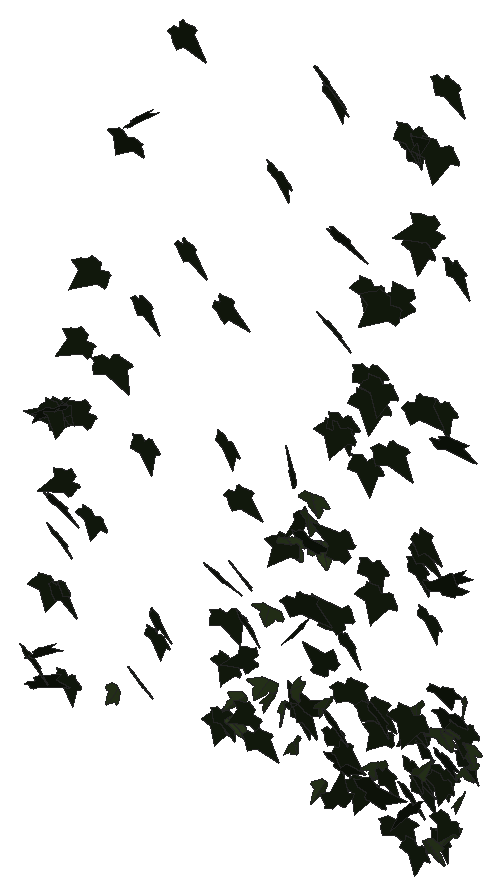
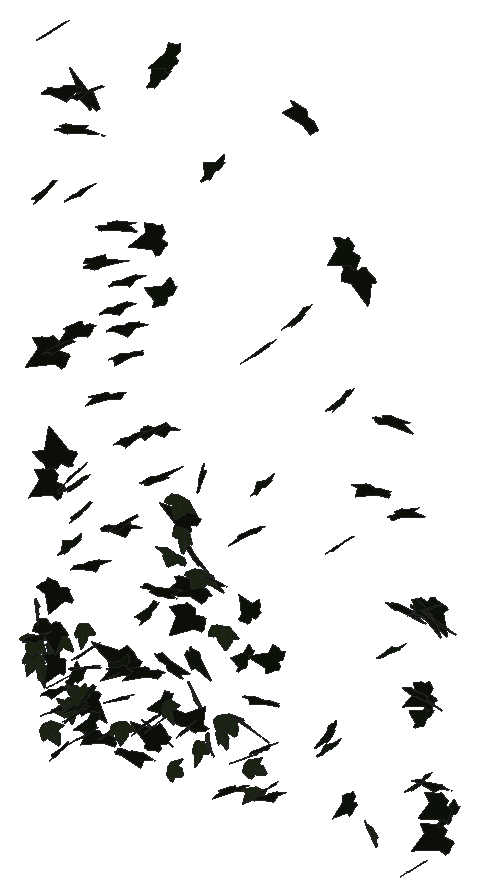
# SketchUp Ruby script. Lengths in inches.
U = 1.inch
M = Sketchup.active_model
def pt(a) = Geom::Point3d.new(a.map { |v| v * U })
def face(e, loops, mat)
  f = e.add_face(loops[0].map { |a| pt(a) })
  loops[1..].each { |l| e.add_face(l.map { |a| pt(a) }).erase! }
  f.material = f.back_material = mat if mat
  f
end
# faces: each face lists its corners as indices into pts; further lists are holes
def faces(e, pts, list, mat = nil) = list.each { |f| face(e, (f[0].is_a?(Array) ? f : [f]).map { |l| l.map { |i| pts[i] } }, mat) }
# xy, xz, yz: faces in a plane at the given z, y or x. An outline is a flat list of corners, or four numbers for a rectangle; further outlines are holes
def ring(l) = l.size == 4 ? [[l[0], l[1]], [l[2], l[1]], [l[2], l[3]], [l[0], l[3]]] : l.each_slice(2).to_a
def flat(e, list, mat, &to3) = list.each { |f| face(e, (f[0].is_a?(Array) ? f : [f]).map { |l| ring(l).map { |u, v| to3.(u, v) } }, mat) }
def xy(e, z, list, mat = nil) = flat(e, list, mat) { |x, y| [x, y, z] }
def xz(e, y, list, mat = nil) = flat(e, list, mat) { |x, z| [x, y, z] }
def yz(e, x, list, mat = nil) = flat(e, list, mat) { |y, z| [x, y, z] }
def lines(e, pts, list) = list.each { |a, b| e.add_line(pt(pts[a]), pt(pts[b])) }
# prism: a flat outline (further loops are holes) pulled along v
def prism(e, loops, v, mat = nil)
  f = face(e, loops, mat); d = Geom::Vector3d.new(v.map { |x| x * U })
  f.pushpull(f.normal.samedirection?(d) ? d.length : -d.length)
end
def box(e, o, s, mat = nil) = prism(e, [[o, [o[0] + s[0], o[1], o[2]], [o[0] + s[0], o[1] + s[1], o[2]], [o[0], o[1] + s[1], o[2]]]], [0, 0, s[2]], mat)
def at(x, y, z, deg = 0) = Geom::Transformation.translation(pt([x, y, z])) * Geom::Transformation.rotation(ORIGIN, Z_AXIS, deg.degrees)
def axes(o, x, y, z) = Geom::Transformation.new([*x, 0, *y, 0, *z, 0, *pt(o).to_a, 1])
def part(name) = M.definitions.add(name)
# library, detail: a bought-in or finely detailed component or shape, given as its bounding box
def library(name, o, s) = part(name).tap { |d| box(d.entities, o, s) }
def detail(e, o, s) = box(e.add_group.entities, o, s)
def put(e, d, t, mat = nil) = e.add_instance(d, t).tap { |i| i.material = mat if mat }
def group(e, t, mat = nil) = e.add_group.tap { |g| g.transformation = t; g.material = mat if mat }.entities
root = M.entities
M.materials.add("1026 AP 7946 SUNNY SIDE UP").color = [254, 231, 186]
M.materials.add("efeu1").color = [18, 25, 13]
M.materials.add("efeu2").color = [43, 57, 29]
c1 = part("ivyleaf_9")
p = [[1.54,2.16,1.25],[1.36,2.04,1.19],[-0.21,0.99,0.68],[-0.71,1.11,0.82],[-0.85,0.86,0.67],[-0.8,0.17,0.21],
  [-0.9,-0.01,0.1],[-0.67,-0.16,-0.02],[-0.08,-0.08,-0.05],[-0.03,-0.6,-0.4],[0.65,-0.88,-0.66],[0.83,-0.6,-0.49],
  [1.29,-0.42,-0.43],[1.8125,-0.07,-0.26],[1.21,0.44,0.15]]
faces(c1.entities,p,[[0,1,2,3,4,5,6,7,8,9,10,11,12,13,14]],"efeu1")
c2 = part("ivyleaf_10")
p = [[0,0.5,-0.03],[-0.0625,2.02,-0.43],[-0.19,2.01,-0.46],[-0.54,1.05,-0.29],[-0.52,0.625,-0.18],[-0.83,0.76,-0.28],
  [-1.16,0.64,-0.33],[-1.15,0.33,-0.24],[-0.77,-0.39,0.02],[-0.3,-0.51,0.16],[0.04,-0.48,0.23],[-0.02,2.01,-0.4375],
  [-0.06,2.01,-0.43],[0.04,-0.49,0.23],[0.67,-0.49,0.14],[1.38,0.36,-0.2],[1.375,0.51,-0.24],[0.81,0.65,-0.19],
  [0.62,0.59,-0.15],[0.6,1.09,-0.28],[0.5,1.23,-0.31]]
faces(c2.entities,p,[[0,1,2,3,4,5,6,7,8,9,10],[11,12,0,13,14,15,16,17,18,19,20]],"efeu2")
put(root,c1,axes([99.83,212.1875,300.87],[-0.58359,0.05469,0.08508],[-0.13611,-0.0259,-0.38471],[-0.07485,-0.37927,0.03627]),"1026 AP 7946 SUNNY SIDE UP")
put(root,c1,axes([99.74,211.14,304.6],[-0.03122,0.37574,-0.19386],[-0.0981,-0.18665,-0.4002],[-0.7049,0.00934,0.06428]),"1026 AP 7946 SUNNY SIDE UP")
put(root,c1,axes([99.41,211.6,296.37],[-0.47274,-0.25055,-0.10343],[0.23864,-0.02256,-0.38449],[0.38608,-0.29284,0.11101]),"1026 AP 7946 SUNNY SIDE UP")
put(root,c1,axes([100.02,211.4,304.22],[-0.5025,0.19094,0.23112],[-0.35056,0.07026,-0.37301],[-0.33673,-0.35808,0.04344]),"1026 AP 7946 SUNNY SIDE UP")
put(root,c1,axes([99.85,211.42,304.61],[-0.25238,0.37371,-0.02021],[-0.03373,-0.03339,-0.42979],[-0.63478,-0.14681,0.03087]),"1026 AP 7946 SUNNY SIDE UP")
put(root,c1,axes([99.59,211.3125,300.41],[0.62802,-0.14559,0.00543],[-0.01208,-0.03703,-0.4243],[0.24713,0.36817,-0.03454]),"1026 AP 7946 SUNNY SIDE UP")
put(root,c1,axes([99.82,211.47,304.43],[-0.215,-0.37216,0.08626],[0.03995,-0.09744,-0.41847],[0.64696,-0.11766,0.0545]),"1026 AP 7946 SUNNY SIDE UP")
put(root,c1,axes([99.62,209.84,293.97],[0.27049,-0.33274,0.17999],[0.10805,-0.16065,-0.39704],[0.62696,0.17124,-0.00923]),"1026 AP 7946 SUNNY SIDE UP")
put(root,c1,axes([99.73,211.52,296.33],[0.28251,-0.33441,-0.08104],[-0.03589,0.06913,-0.39873],[0.57933,0.16736,0.01482]),"1026 AP 7946 SUNNY SIDE UP")
put(root,c1,axes([99.99,211.83,292.19],[-0.00976,-0.3614,0.06],[0.00416,-0.0608,-0.38778],[0.62208,-0.00526,0.00354]),"1026 AP 7946 SUNNY SIDE UP")
put(root,c1,axes([100.01,209.74,294.23],[0.3581,0.22641,0.29105],[0.26971,0.21835,-0.3272],[-0.53232,0.26294,0.03001]),"1026 AP 7946 SUNNY SIDE UP")
put(root,c1,axes([99.94,209.9375,292.86],[0.47353,0.22274,0.23306],[0.29589,0.12583,-0.38028],[-0.434,0.32881,-0.00498]),"1026 AP 7946 SUNNY SIDE UP")
put(root,c1,axes([99.97,211.08,299.05],[0.21611,-0.29973,0.20391],[0.14768,-0.17645,-0.34057],[0.54667,0.16616,0.0114]),"1026 AP 7946 SUNNY SIDE UP")
put(root,c1,axes([100.86,211.91,304.47],[-0.6169,-0.0056,0.05529],[-0.08298,-0.04357,-0.4021],[0.01796,-0.39358,0.0414]),"1026 AP 7946 SUNNY SIDE UP")
put(root,c1,axes([101.42,211.07,308.3],[-0.41103,-0.22863,0.2234],[-0.23064,-0.16298,-0.35799],[0.44012,-0.29893,0.02103]),"1026 AP 7946 SUNNY SIDE UP")
put(root,c1,axes([102.57,210.5,312.17],[-0.60558,-0.15883,0.07956],[-0.0951,-0.05776,-0.42841],[0.26158,-0.38871,0.02845]),"1026 AP 7946 SUNNY SIDE UP")
put(root,c1,axes([102.45,210.375,300.97],[-0.15504,-0.33744,0.18943],[0.06958,-0.20044,-0.352],[0.60168,-0.06377,0.08952]),"1026 AP 7946 SUNNY SIDE UP")
put(root,c2,axes([102.84,211.22,292.86],[0.40782,-0.25476,-0.08],[-0.09027,0.05029,-0.37421],[0.40826,0.26561,-0.00283]),"1026 AP 7946 SUNNY SIDE UP")
put(root,c1,axes([103.41,210.25,308.45],[-0.15653,-0.3069,-0.27978],[0.34611,0.19373,-0.30951],[0.54139,-0.21258,0.11698]),"1026 AP 7946 SUNNY SIDE UP")
put(root,c1,axes([104,210.53,318.68],[0.39544,0.08936,-0.3623],[-0.50401,-0.14716,-0.27512],[-0.26908,0.40698,-0.01712]),"1026 AP 7946 SUNNY SIDE UP")
put(root,c1,axes([103.65,211.38,293.86],[0.49089,-0.18472,-0.10069],[-0.13516,0.04458,-0.3734],[0.29869,0.32376,-0.00349]),"1026 AP 7946 SUNNY SIDE UP")
put(root,c1,axes([104.34,210.55,319.54],[0.29308,0.24023,0.3354],[0.23971,0.28873,-0.309],[-0.58745,0.23767,0.04124]),"1026 AP 7946 SUNNY SIDE UP")
put(root,c1,axes([104.73,211.33,296.88],[0.401,-0.25528,-0.1437],[-0.16759,0.08854,-0.37102],[0.42445,0.27614,-0.01073]),"1026 AP 7946 SUNNY SIDE UP")
put(root,c1,axes([104.86,211.41,295.99],[-0.00841,-0.34617,0.16765],[0.05573,-0.16446,-0.35587],[0.6002,0.01042,0.03539]),"1026 AP 7946 SUNNY SIDE UP")
put(root,c1,axes([105.06,210.39,305.26],[0.02898,-0.41221,0.02212],[-0.00057,-0.02385,-0.42522],[0.64924,0.01838,-0.00136]),"1026 AP 7946 SUNNY SIDE UP")
put(root,c1,axes([105.22,209.9,311.93],[0.32539,-0.37606,-0.06268],[-0.0472,0.05049,-0.4419],[0.59662,0.20909,-0.00078]),"1026 AP 7946 SUNNY SIDE UP")
put(root,c1,axes([107.09,210.11,324.84],[-0.019,-0.13716,-0.46068],[0.71861,0.08836,-0.04019],[0.151,-0.43773,0.13332]),"1026 AP 7946 SUNNY SIDE UP")
put(root,c1,axes([107.4,209.93,315.23],[0.38057,-0.35202,-0.12857],[-0.08086,0.11349,-0.4389],[0.58063,0.24653,0.02315]),"1026 AP 7946 SUNNY SIDE UP")
put(root,c1,axes([107.25,211.89,299.55],[0.40144,-0.22967,0.20304],[0.25758,-0.11396,-0.35375],[0.40173,0.30258,0.02393]),"1026 AP 7946 SUNNY SIDE UP")
put(root,c1,axes([107.78,211.875,292.96],[-0.25651,-0.32362,0.03608],[-0.00352,-0.04011,-0.37322],[0.51213,-0.16237,0.0155]),"1026 AP 7946 SUNNY SIDE UP")
put(root,c1,axes([107.78,212.31,295.38],[-0.20276,-0.32363,0.12616],[-0.02449,-0.12708,-0.35824],[0.54457,-0.12621,0.03086]),"1026 AP 7946 SUNNY SIDE UP")
put(root,c1,axes([107.75,211.9,293.31],[0.12283,-0.34841,-0.08176],[-0.00623,0.07836,-0.36714],[0.56116,0.07713,0.01382]),"1026 AP 7946 SUNNY SIDE UP")
put(root,c1,axes([107.78,212.17,297.64],[-0.18146,-0.31815,-0.20509],[0.36579,0.10078,-0.30706],[0.46117,-0.20513,0.16286]),"1026 AP 7946 SUNNY SIDE UP")
put(root,c2,axes([108.55,212.05,294.15],[-0.10016,-0.19594,0.33649],[-0.08152,-0.32475,-0.2123],[0.59485,-0.0775,0.02757]),"1026 AP 7946 SUNNY SIDE UP")
put(root,c2,axes([108.23,211.92,293],[0.20225,0.27919,0.21179],[0.16669,0.17533,-0.31504],[-0.51751,0.16558,-0.0187]),"1026 AP 7946 SUNNY SIDE UP")
put(root,c1,axes([109.13,212.03,296.13],[-0.52546,0.15071,0.08465],[-0.14384,-0.00637,-0.37516],[-0.22764,-0.34387,0.04165]),"1026 AP 7946 SUNNY SIDE UP")
put(root,c1,axes([109.48,211.625,293.92],[-0.37227,-0.15516,0.27387],[-0.14877,-0.28349,-0.25807],[0.46182,-0.21639,0.13763]),"1026 AP 7946 SUNNY SIDE UP")
put(root,c1,axes([109.11,210.53,306.62],[0.05076,-0.36475,0.21302],[0.04929,-0.20679,-0.37826],[0.65906,0.04356,0.01188]),"1026 AP 7946 SUNNY SIDE UP")
put(root,c1,axes([109.18,210.09,313.14],[0.40116,-0.27524,-0.23936],[-0.09786,0.24492,-0.37036],[0.55625,0.24159,0.10747]),"1026 AP 7946 SUNNY SIDE UP")
put(root,c1,axes([109.39,211.97,292.81],[0.13035,-0.30689,-0.22335],[0.10044,0.22861,-0.30937],[0.58063,0.02935,0.10366]),"1026 AP 7946 SUNNY SIDE UP")
put(root,c1,axes([109.37,210.9375,300.57],[0.02789,-0.19761,0.36281],[0.23856,-0.32462,-0.19679],[0.59013,0.14057,0.06241]),"1026 AP 7946 SUNNY SIDE UP")
put(root,c1,axes([109.54,210.61,304.44],[0.22612,-0.31057,-0.24555],[0.00137,0.25239,-0.33929],[0.61391,0.11383,0.0912]),"1026 AP 7946 SUNNY SIDE UP")
put(root,c1,axes([109.48,211.11,298.49],[0.27876,-0.3173,0.16834],[0.08244,-0.15934,-0.37417],[0.55642,0.18257,-0.0289]),"1026 AP 7946 SUNNY SIDE UP")
put(root,c2,axes([110.23,211.61,295.61],[-0.4089,-0.23406,0.18806],[-0.11309,-0.18752,-0.35179],[0.45416,-0.25743,0.08172]),"1026 AP 7946 SUNNY SIDE UP")
put(root,c2,axes([110.35,211.74,295],[0.00054,-0.36267,0.0881],[0.0017,-0.08757,-0.37413],[0.58665,0.00059,0.001]),"1026 AP 7946 SUNNY SIDE UP")
put(root,c2,axes([110.84,211.05,299.4],[-0.58734,-0.03665,0.0962],[-0.13507,-0.07059,-0.38209],[0.08205,-0.37855,0.05962]),"1026 AP 7946 SUNNY SIDE UP")
put(root,c2,axes([110.72,212.09,294.54],[0.31309,-0.2741,0.18309],[0.17542,-0.14051,-0.34977],[0.48421,0.22813,0.00832]),"1026 AP 7946 SUNNY SIDE UP")
put(root,c1,axes([111.16,211.83,302.17],[-0.59097,-0.10776,-0.06398],[0.11804,-0.04132,-0.39831],[0.15533,-0.37859,0.05926]),"1026 AP 7946 SUNNY SIDE UP")
put(root,c2,axes([111.21,211.88,302.27],[-0.54863,-0.12554,-0.14393],[0.2538,-0.05246,-0.3689],[0.14939,-0.3719,0.09815]),"1026 AP 7946 SUNNY SIDE UP")
put(root,c1,axes([111.625,212.09,298.45],[-0.34465,0.27765,-0.17559],[0.12922,-0.15361,-0.36421],[-0.49706,-0.23245,0.02706]),"1026 AP 7946 SUNNY SIDE UP")
put(root,c1,axes([111.7,212.13,303.43],[-0.49144,0.17625,-0.17962],[0.21752,-0.11077,-0.36935],[-0.32482,-0.34083,0.02442]),"1026 AP 7946 SUNNY SIDE UP")
put(root,c1,axes([111.95,211.88,294.88],[0.33035,0.03584,0.34767],[-0.50458,0.14947,0.19044],[-0.17268,-0.36817,0.10863]),"1026 AP 7946 SUNNY SIDE UP")
put(root,c2,axes([111.86,211.29,293.61],[-0.06529,-0.35415,-0.17677],[0.06426,0.1657,-0.36584],[0.61406,-0.055,0.01949]),"1026 AP 7946 SUNNY SIDE UP")
put(root,c2,axes([111.7,211.57,295.89],[0.23162,-0.27798,-0.25158],[0.2512,-0.18744,0.32006],[-0.52298,-0.21315,0.04231]),"1026 AP 7946 SUNNY SIDE UP")
put(root,c1,axes([111.78,211.83,294.85],[0.11274,-0.36514,0.0289],[-0.00813,-0.0317,-0.38336],[0.57604,0.07101,-0.01107]),"1026 AP 7946 SUNNY SIDE UP")
put(root,c1,axes([112.22,210.82,305.88],[-0.03748,-0.22222,0.37253],[0.05916,0.36092,0.23236],[-0.66646,0.04454,-0.00032]),"1026 AP 7946 SUNNY SIDE UP")
put(root,c1,axes([111.87,211.85,294.875],[0.1984,-0.33517,-0.111],[-0.06656,0.09715,-0.36834],[0.54865,0.13299,-0.00455]),"1026 AP 7946 SUNNY SIDE UP")
put(root,c1,axes([111.97,211.49,299.92],[0.58575,0.16081,0.03101],[0.0679,-0.02678,-0.41595],[-0.24786,0.3727,-0.04067]),"1026 AP 7946 SUNNY SIDE UP")
put(root,c2,axes([112.36,211.72,303.79],[-0.54421,0.19018,0.07752],[-0.13723,-0.00589,-0.40405],[-0.29016,-0.35391,0.04571]),"1026 AP 7946 SUNNY SIDE UP")
put(root,c1,axes([112.26,209.8,320.3],[0.12992,-0.38592,0.24713],[0.11186,-0.23208,-0.40752],[0.70754,0.10756,0.01905]),"1026 AP 7946 SUNNY SIDE UP")
put(root,c1,axes([113.15,211.8,297.27],[-0.07024,0.14374,0.39196],[-0.42008,0.27717,-0.13887],[-0.48062,-0.26327,0.0641]),"1026 AP 7946 SUNNY SIDE UP")
put(root,c2,axes([112.8,211.38,305.03],[-0.63021,0.03903,-0.0285],[0.03772,-0.04017,-0.41328],[-0.06531,-0.39975,0.03636]),"1026 AP 7946 SUNNY SIDE UP")
put(root,c2,axes([112.88,212.11,295.51],[-0.04831,-0.36778,0.06425],[-0.00477,-0.06442,-0.38057],[0.58709,-0.03079,0.00219]),"1026 AP 7946 SUNNY SIDE UP")
put(root,c1,axes([112.6,210.6,300.6875],[-0.03897,-0.08414,-0.43849],[0.43178,0.32642,-0.08113],[0.52725,-0.27354,0.03403]),"1026 AP 7946 SUNNY SIDE UP")
put(root,c2,axes([112.84,211.81,302.65],[0.58567,0.04095,0.15584],[0.24081,-0.0152,-0.38491],[-0.0506,0.40164,-0.02808]),"1026 AP 7946 SUNNY SIDE UP")
put(root,c2,axes([113.22,211.39,292.11],[-0.04184,-0.24833,0.31173],[0.0972,-0.30355,-0.25164],[0.60952,0.03136,0.06153]),"1026 AP 7946 SUNNY SIDE UP")
put(root,c1,axes([113,210.54,303.51],[0.16638,-0.13308,0.37409],[0.4676,-0.21391,-0.17093],[0.39053,0.31281,0.04528]),"1026 AP 7946 SUNNY SIDE UP")
put(root,c1,axes([113.36,211.6,295.26],[0.37909,-0.31113,0.0561],[0.02342,-0.05945,-0.40506],[0.4966,0.24031,-0.02372]),"1026 AP 7946 SUNNY SIDE UP")
put(root,c1,axes([113.49,211.7,294.52],[0.24299,-0.34122,-0.1354],[-0.05789,0.12534,-0.38475],[0.57094,0.15793,0.01862]),"1026 AP 7946 SUNNY SIDE UP")
put(root,c1,axes([113.64,212.1875,308.5],[-0.0132,-0.43438,-0.03615],[-0.00099,0.03264,-0.44738],[0.68494,-0.00833,-0.00135]),"1026 AP 7946 SUNNY SIDE UP")
put(root,c1,axes([113.83,211.71,308.34],[-0.40622,-0.32279,-0.02529],[0.08417,-0.01396,-0.42283],[0.5018,-0.25896,0.05045]),"1026 AP 7946 SUNNY SIDE UP")
put(root,c1,axes([114.45,211.14,300.1],[-0.5579,-0.17923,-0.13117],[-0.2044,-0.02156,0.40755],[-0.27765,0.376,-0.03645]),"1026 AP 7946 SUNNY SIDE UP")
put(root,c1,axes([113.75,211.55,317.33],[0.64858,-0.167,0.09296],[0.10531,-0.07633,-0.45657],[0.28004,0.41548,-0.04361]),"1026 AP 7946 SUNNY SIDE UP")
put(root,c1,axes([113.77,211.57,293.26],[0.18555,-0.13092,0.3712],[0.44868,-0.22294,-0.18066],[0.40422,0.30755,0.03013]),"1026 AP 7946 SUNNY SIDE UP")
put(root,c1,axes([114.07,211.9,296.72],[0.04122,-0.27406,-0.3065],[0.21995,0.28436,-0.25684],[0.5949,-0.08615,0.1162]),"1026 AP 7946 SUNNY SIDE UP")
put(root,c1,axes([114.23,211.34,294.16],[0.30009,-0.24696,-0.26129],[-0.12619,0.24886,-0.31213],[0.54051,0.19521,0.07219]),"1026 AP 7946 SUNNY SIDE UP")
put(root,c1,axes([114.0625,210.22,325.3],[0.53625,-0.33183,0.02125],[-0.01195,-0.04,-0.48919],[0.52283,0.33943,-0.03297]),"1026 AP 7946 SUNNY SIDE UP")
put(root,c1,axes([114.33,211.45,299.21],[0.28727,-0.36102,0.06595],[0.01337,-0.06962,-0.41653],[0.57694,0.18137,-0.02318]),"1026 AP 7946 SUNNY SIDE UP")
put(root,c1,axes([114.29,210.44,313.91],[0.28648,-0.34292,0.22918],[0.20711,-0.18355,-0.40021],[0.61021,0.22329,0.02824]),"1026 AP 7946 SUNNY SIDE UP")
put(root,c1,axes([114.56,210.51,324.22],[0.06277,-0.35751,0.31546],[0.13139,-0.29911,-0.37028],[0.73053,0.08451,0.03949]),"1026 AP 7946 SUNNY SIDE UP")
put(root,c1,axes([115.08,210.07,292.61],[-0.55602,0.22203,-0.06799],[-0.05989,0.06539,0.42904],[0.35983,0.35396,-0.03365]),"1026 AP 7946 SUNNY SIDE UP")
put(root,c1,axes([115.01,211.95,292.5],[-0.51284,-0.22727,-0.09998],[0.14336,0.03641,-0.40871],[0.36031,-0.33796,0.02031]),"1026 AP 7946 SUNNY SIDE UP")
put(root,c1,axes([115.6,209.9,304.37],[-0.29366,-0.42523,-0.02972],[-0.04224,-0.01705,0.47801],[-0.6686,0.18785,-0.01714]),"1026 AP 7946 SUNNY SIDE UP")
put(root,c1,axes([115.21,212.125,315.09],[-0.24729,-0.39985,0.05275],[-0.0035,-0.05654,-0.44256],[0.63431,-0.15619,0.01813]),"1026 AP 7946 SUNNY SIDE UP")
put(root,c1,axes([115.25,211.67,307.37],[-0.0939,-0.42883,-0.03959],[0.00493,0.0359,-0.44583],[0.67665,-0.05977,-0.00224]),"1026 AP 7946 SUNNY SIDE UP")
put(root,c2,axes([115.5,212.02,293.58],[-0.27638,-0.32182,0.00182],[0.02079,-0.01132,-0.37742],[0.50564,-0.17544,0.01652]),"1026 AP 7946 SUNNY SIDE UP")
put(root,c1,axes([115.21,211.9,311.43],[-0.04033,-0.39998,-0.14106],[0.10387,0.12944,-0.40829],[0.65544,-0.04513,0.05602]),"1026 AP 7946 SUNNY SIDE UP")
put(root,c1,axes([115.58,212.31,294.98],[-0.32537,-0.26657,0.16479],[-0.04262,-0.1777,-0.33904],[0.48821,-0.19318,0.08023]),"1026 AP 7946 SUNNY SIDE UP")
put(root,c1,axes([115.35,211.83,296.33],[0.06418,-0.28791,-0.29316],[0.15763,0.2827,-0.2798],[0.61484,-0.04243,0.10234]),"1026 AP 7946 SUNNY SIDE UP")
put(root,c1,axes([115.77,211.41,303.01],[0.02646,-0.42375,-0.04791],[-0.01272,0.04381,-0.43658],[0.66978,0.01757,-0.0064]),"1026 AP 7946 SUNNY SIDE UP")
put(root,c1,axes([115.69,211.78,296.1875],[0.13289,-0.34405,0.1998],[0.11132,-0.18395,-0.36536],[0.61249,0.10808,0.02305]),"1026 AP 7946 SUNNY SIDE UP")
put(root,c1,axes([115.88,212.02,293.33],[0.22122,-0.33606,-0.07929],[-0.02973,0.07342,-0.37473],[0.54062,0.14155,0.01184]),"1026 AP 7946 SUNNY SIDE UP")
put(root,c1,axes([116.64,210.81,302.25],[-0.39753,-0.34947,-0.01892],[0.04657,-0.00124,-0.44363],[0.54814,-0.25334,0.02397]),"1026 AP 7946 SUNNY SIDE UP")
put(root,c1,axes([117.05,211.98,315.16],[-0.36742,-0.05636,0.37232],[-0.48248,-0.20392,-0.23812],[0.31398,-0.3793,0.06978]),"1026 AP 7946 SUNNY SIDE UP")
put(root,c1,axes([116.8,210.11,311.45],[-0.28223,-0.42677,-0.02719],[0.04547,0.01381,-0.47638],[0.67058,-0.18055,0.02086]),"1026 AP 7946 SUNNY SIDE UP")
put(root,c1,axes([116.7,211.22,308.69],[0.06969,-0.36897,-0.24854],[0.16765,0.24222,-0.3632],[0.67076,-0.02221,0.1166]),"1026 AP 7946 SUNNY SIDE UP")
put(root,c1,axes([117.24,210.19,312.21],[-0.23023,-0.40261,0.03031],[-0.00395,-0.03282,-0.44144],[0.63501,-0.14618,0.00825]),"1026 AP 7946 SUNNY SIDE UP")
put(root,c1,axes([117.04,211.83,293.15],[0.40285,-0.3053,0.03687],[0.00806,-0.04459,-0.41007],[0.4836,0.25507,-0.02388]),"1026 AP 7946 SUNNY SIDE UP")
put(root,c1,axes([117.57,210.13,316.01],[-0.53106,-0.28057,0.17339],[-0.15452,-0.14611,-0.45067],[0.49205,-0.34869,0.04561]),"1026 AP 7946 SUNNY SIDE UP")
put(root,c1,axes([117.5625,212.17,295.76],[-0.43297,-0.19545,0.15569],[-0.07526,-0.18135,-0.3301],[0.38221,-0.25711,0.11136]),"1026 AP 7946 SUNNY SIDE UP")
put(root,c1,axes([117.32,211.78,296.52],[0.22264,-0.341,-0.09072],[0.00292,0.09356,-0.37795],[0.55301,0.13679,0.03852]),"1026 AP 7946 SUNNY SIDE UP")
put(root,c1,axes([117.32,211,292.11],[-0.14108,-0.2399,-0.32119],[0.34981,0.23117,-0.24894],[0.5081,-0.22576,0.0822]),"1026 AP 7946 SUNNY SIDE UP")
put(root,c1,axes([117.38,212.19,303.28],[0.17972,-0.38489,0.03089],[-0.00392,-0.03428,-0.41364],[0.6073,0.11368,-0.01181]),"1026 AP 7946 SUNNY SIDE UP")
put(root,c1,axes([117.38,211.83,294.36],[0.19632,-0.34331,0.07138],[0.01661,-0.0719,-0.37647],[0.55107,0.12447,-0.01408]),"1026 AP 7946 SUNNY SIDE UP")
put(root,c1,axes([117.51,211.8,323.13],[-0.04979,-0.4719,-0.02818],[0.06496,0.02187,-0.48539],[0.74018,-0.03366,0.0407]),"1026 AP 7946 SUNNY SIDE UP")
put(root,c1,axes([117.52,211.88,294.05],[0.38155,-0.27184,-0.07559],[-0.04847,0.06858,-0.37429],[0.43944,0.24359,0.02434]),"1026 AP 7946 SUNNY SIDE UP")
put(root,c2,axes([117.85,211.56,297.23],[-0.12039,-0.36471,-0.10173],[0.06155,0.09044,-0.38288],[0.59008,-0.08385,0.01918]),"1026 AP 7946 SUNNY SIDE UP")
put(root,c1,axes([117.48,211.51,322.46],[-0.09631,0.17412,0.45081],[0.31482,-0.3887,0.18636],[0.66871,0.20807,-0.02281]),"1026 AP 7946 SUNNY SIDE UP")
put(root,c1,axes([117.73,212.2,295.12],[-0.10453,-0.20366,0.33611],[0.07961,-0.33398,-0.20538],[0.60105,0.00882,0.08566]),"1026 AP 7946 SUNNY SIDE UP")
put(root,c1,axes([117.69,212.15,293.52],[0.0926,-0.37804,-0.06332],[0.01266,0.06123,-0.3934],[0.60157,0.0569,0.01803]),"1026 AP 7946 SUNNY SIDE UP")
put(root,c2,axes([117.86,211.74,294.05],[-0.10398,-0.31432,0.22651],[0.04922,0.21976,0.33196],[-0.60277,0.07217,-0.01197]),"1026 AP 7946 SUNNY SIDE UP")
put(root,c1,axes([117.91,211.79,318.17],[-0.10529,-0.42357,0.11176],[-0.03122,-0.10913,-0.44241],[0.68777,-0.0698,-0.00298]),"1026 AP 7946 SUNNY SIDE UP")
put(root,c1,axes([117.52,208.92,294.4],[0.19185,-0.04363,0.46627],[0.58734,-0.25805,-0.1308],[0.40838,0.39163,-0.03093]),"1026 AP 7946 SUNNY SIDE UP")
put(root,c1,axes([117.91,211.78,304.88],[0.30298,-0.30849,-0.24364],[-0.15517,0.21448,-0.37256],[0.58947,0.21502,0.02716]),"1026 AP 7946 SUNNY SIDE UP")
put(root,c1,axes([117.84,211.74,304.33],[0.31838,-0.33469,-0.11675],[0.00369,0.12976,-0.39635],[0.55465,0.19125,0.06966]),"1026 AP 7946 SUNNY SIDE UP")
put(root,c1,axes([118.43,210.55,293.35],[-0.19203,0.27838,-0.31821],[0.16976,-0.29137,-0.3146],[-0.63333,-0.16251,0.01216]),"1026 AP 7946 SUNNY SIDE UP")
put(root,c1,axes([118.16,212,301.25],[0.06477,-0.36434,0.18611],[0.08575,-0.17707,-0.37744],[0.63514,0.06106,0.03198]),"1026 AP 7946 SUNNY SIDE UP")
put(root,c1,axes([118.26,211.11,311.34],[0.11887,-0.23931,-0.38819],[-0.04875,0.37708,-0.25182],[0.69839,0.06705,0.0485]),"1026 AP 7946 SUNNY SIDE UP")
put(root,c1,axes([118.57,210.7,291.48],[-0.07872,-0.38255,0.12039],[-0.01054,-0.11914,-0.39807],[0.62989,-0.0498,0.00838]),"1026 AP 7946 SUNNY SIDE UP")
put(root,c1,axes([118.54,212.27,310.83],[-0.01494,-0.4218,-0.03485],[0.02439,0.03108,-0.4342],[0.66463,-0.01062,0.01515]),"1026 AP 7946 SUNNY SIDE UP")
put(root,c1,axes([118.58,212.17,291.39],[0.11606,-0.34465,0.06832],[0.00556,-0.06903,-0.36334],[0.55243,0.0731,-0.0107]),"1026 AP 7946 SUNNY SIDE UP")
put(root,c1,axes([118.72,212.23,294.33],[-0.10944,-0.36511,-0.06422],[0.04775,0.05548,-0.38207],[0.57991,-0.07347,0.01934]),"1026 AP 7946 SUNNY SIDE UP")
put(root,c1,axes([118.83,211.83,322.8125],[-0.38313,-0.40906,-0.05111],[0.06621,0.02991,-0.48986],[0.6441,-0.2464,0.01995]),"1026 AP 7946 SUNNY SIDE UP")
put(root,c1,axes([119.17,212.01,297.14],[0.39785,0.14089,-0.26445],[-0.34998,-0.12953,-0.29908],[-0.30088,0.33696,-0.00179]),"1026 AP 7946 SUNNY SIDE UP")
put(root,c2,axes([119.03,211.7,296.43],[-0.57146,-0.09633,-0.1252],[0.20029,-0.01124,-0.38504],[0.13789,-0.38287,0.04042]),"1026 AP 7946 SUNNY SIDE UP")
put(root,c1,axes([119.0625,211.68,295.4],[0.5769,-0.07562,-0.17475],[-0.27058,0.00035,-0.38456],[0.10822,0.40403,-0.02993]),"1026 AP 7946 SUNNY SIDE UP")
put(root,c1,axes([118.89,212.05,325.77],[0.22024,-0.43422,-0.08759],[0.02182,0.09088,-0.46765],[0.69466,0.13481,0.04246]),"1026 AP 7946 SUNNY SIDE UP")
put(root,c1,axes([119.125,211.63,294.29],[-0.12213,-0.34345,0.13967],[0.00948,-0.14168,-0.36183],[0.58165,-0.06981,0.03523]),"1026 AP 7946 SUNNY SIDE UP")
put(root,c1,axes([119.65,210.41,320.02],[-0.57297,-0.09779,0.25464],[-0.32873,-0.15507,-0.38077],[0.25944,-0.41244,0.0799]),"1026 AP 7946 SUNNY SIDE UP")
put(root,c2,axes([119.45,211.88,292.0625],[-0.20258,-0.32525,0.19004],[-0.07399,-0.18142,-0.36085],[0.58473,-0.13564,0.02017]),"1026 AP 7946 SUNNY SIDE UP")
put(root,c1,axes([119.24,211.4,298.6],[0.53324,0.13606,-0.12574],[-0.15186,-0.08691,-0.37441],[-0.24496,0.35006,-0.0416]),"1026 AP 7946 SUNNY SIDE UP")
put(root,c1,axes([119.57,211.5,292.68],[-0.23483,-0.30163,0.15034],[-0.04168,-0.1505,-0.34524],[0.52641,-0.14647,0.03973]),"1026 AP 7946 SUNNY SIDE UP")
put(root,c1,axes([119.49,211.37,303.6],[0.32081,0.27726,0.28908],[0.27868,0.21583,-0.35317],[-0.55218,0.27001,-0.01028]),"1026 AP 7946 SUNNY SIDE UP")
put(root,c1,axes([119.35,211.36,309.92],[0.68104,0.09488,0.09006],[0.14643,-0.02069,-0.45509],[-0.13957,0.44126,-0.038]),"1026 AP 7946 SUNNY SIDE UP")
put(root,c1,axes([119.71,209.02,298.57],[-0.33465,-0.40117,0.05409],[-0.00034,-0.06178,-0.46728],[0.63666,-0.2109,0.02818]),"1026 AP 7946 SUNNY SIDE UP")
put(root,c1,axes([119.67,212.29,296.59],[-0.17748,-0.36552,-0.03828],[0.03747,0.02934,-0.39366],[0.57617,-0.1145,0.01381]),"1026 AP 7946 SUNNY SIDE UP")
put(root,c1,axes([119.5,211.89,317.72],[0.24948,-0.41269,0.01396],[-0.00926,-0.01928,-0.45542],[0.64932,0.15828,-0.01186]),"1026 AP 7946 SUNNY SIDE UP")
put(root,c2,axes([119.64,210.23,292.21],[-0.39137,0.13112,-0.2851],[0.34433,-0.17445,-0.2883],[-0.33813,-0.32942,0.03642]),"1026 AP 7946 SUNNY SIDE UP")
put(root,c2,axes([119.94,212.02,297.87],[0.2347,-0.33039,-0.11149],[0.00841,0.11793,-0.36904],[0.54568,0.14028,0.05364]),"1026 AP 7946 SUNNY SIDE UP")
put(root,c2,axes([120.11,211.9375,296.04],[-0.56572,0.07626,-0.0881],[0.11387,-0.06886,-0.37562],[-0.14028,-0.36344,0.05039]),"1026 AP 7946 SUNNY SIDE UP")
put(root,c1,axes([119.91,211.99,295.5625],[0.2399,-0.33821,-0.04153],[-0.03175,0.03301,-0.38201],[0.53428,0.15382,-0.00405]),"1026 AP 7946 SUNNY SIDE UP")
put(root,c2,axes([120.29,211.85,295.18],[-0.19106,-0.35224,-0.13926],[0.11892,0.11426,-0.38175],[0.58006,-0.13944,0.03239]),"1026 AP 7946 SUNNY SIDE UP")
put(root,c1,axes([120.1,210.28,303.92],[0.65503,0.12856,0.11315],[-0.1834,0.0097,0.44706],[0.19146,-0.43052,0.04111]),"1026 AP 7946 SUNNY SIDE UP")
put(root,c2,axes([120.48,211.12,294.21],[0.06769,-0.36947,-0.00624],[-0.00638,0.00351,-0.38317],[0.58096,0.04309,-0.00348]),"1026 AP 7946 SUNNY SIDE UP")
